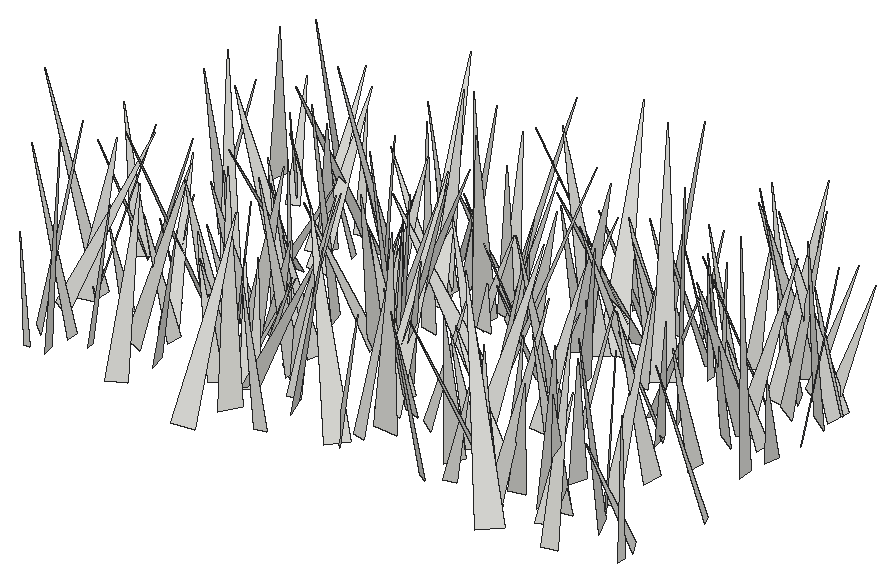
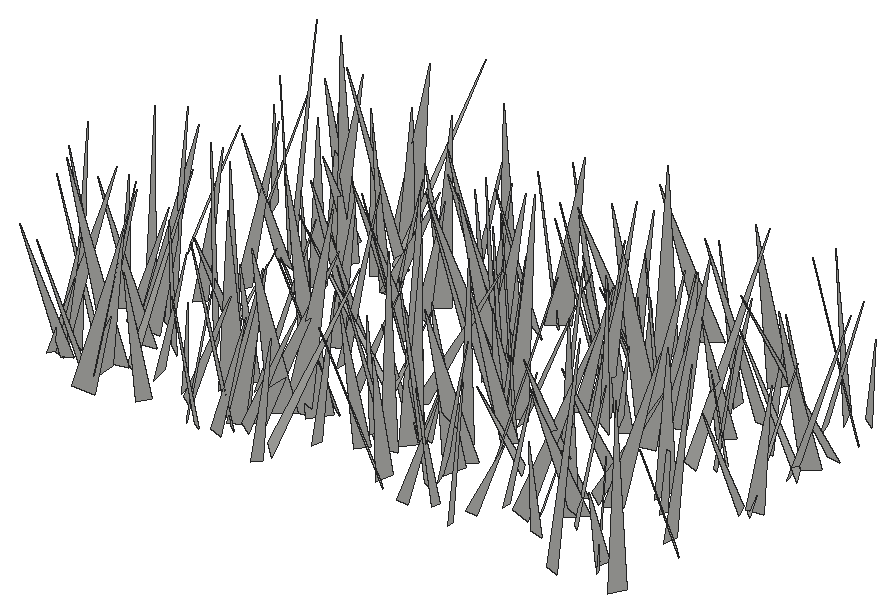
# SketchUp Ruby script. Lengths in inches.
U = 1.inch
M = Sketchup.active_model
def pt(a) = Geom::Point3d.new(a.map { |v| v * U })
def face(e, loops, mat)
  f = e.add_face(loops[0].map { |a| pt(a) })
  loops[1..].each { |l| e.add_face(l.map { |a| pt(a) }).erase! }
  f.material = f.back_material = mat if mat
  f
end
# faces: each face lists its corners as indices into pts; further lists are holes
def faces(e, pts, list, mat = nil) = list.each { |f| face(e, (f[0].is_a?(Array) ? f : [f]).map { |l| l.map { |i| pts[i] } }, mat) }
# xy, xz, yz: faces in a plane at the given z, y or x. An outline is a flat list of corners, or four numbers for a rectangle; further outlines are holes
def ring(l) = l.size == 4 ? [[l[0], l[1]], [l[2], l[1]], [l[2], l[3]], [l[0], l[3]]] : l.each_slice(2).to_a
def flat(e, list, mat, &to3) = list.each { |f| face(e, (f[0].is_a?(Array) ? f : [f]).map { |l| ring(l).map { |u, v| to3.(u, v) } }, mat) }
def xy(e, z, list, mat = nil) = flat(e, list, mat) { |x, y| [x, y, z] }
def xz(e, y, list, mat = nil) = flat(e, list, mat) { |x, z| [x, y, z] }
def yz(e, x, list, mat = nil) = flat(e, list, mat) { |y, z| [x, y, z] }
def lines(e, pts, list) = list.each { |a, b| e.add_line(pt(pts[a]), pt(pts[b])) }
# prism: a flat outline (further loops are holes) pulled along v
def prism(e, loops, v, mat = nil)
  f = face(e, loops, mat); d = Geom::Vector3d.new(v.map { |x| x * U })
  f.pushpull(f.normal.samedirection?(d) ? d.length : -d.length)
end
def box(e, o, s, mat = nil) = prism(e, [[o, [o[0] + s[0], o[1], o[2]], [o[0] + s[0], o[1] + s[1], o[2]], [o[0], o[1] + s[1], o[2]]]], [0, 0, s[2]], mat)
def at(x, y, z, deg = 0) = Geom::Transformation.translation(pt([x, y, z])) * Geom::Transformation.rotation(ORIGIN, Z_AXIS, deg.degrees)
def axes(o, x, y, z) = Geom::Transformation.new([*x, 0, *y, 0, *z, 0, *pt(o).to_a, 1])
def part(name) = M.definitions.add(name)
# library, detail: a bought-in or finely detailed component or shape, given as its bounding box
def library(name, o, s) = part(name).tap { |d| box(d.entities, o, s) }
def detail(e, o, s) = box(e.add_group.entities, o, s)
def put(e, d, t, mat = nil) = e.add_instance(d, t).tap { |i| i.material = mat if mat }
def group(e, t, mat = nil) = e.add_group.tap { |g| g.transformation = t; g.material = mat if mat }.entities
root = M.entities
c1 = part("fur_instance\#9")
p = [[0.8125,0,1.79],[0.67,-0.02,1.48],[0,-0.11,0],[0,0.11,0]]
faces(c1.entities,p,[[0,1,2,3]])
put(root,c1,axes([470.13,224.69,-21.66],[-2.04424,6.85145,0.72305],[6.79433,2.1298,-0.97223],[1.1412,-0.40704,7.08351]))
put(root,c1,axes([456.1,226.65,-21.66],[1.10778,3.32388,1.25845],[3.28018,-1.46364,0.97838],[-1.36832,-0.8177,3.36424]))
put(root,c1,axes([491.39,229.9,-21.66],[-5.30348,-5.59312,0.1785],[-5.55783,5.29332,0.73008],[0.65218,-0.37354,7.67313]))
put(root,c1,axes([474.1875,227.32,-21.66],[-0.90978,-4.59674,2.27002],[-5.08569,0.51819,-0.98893],[-0.64715,2.39002,4.58036]))
put(root,c1,axes([463.36,226.53,-21.66],[-4.06355,5.05875,1.67662],[5.05755,4.32523,-0.79246],[1.68023,-0.78477,6.44014]))
put(root,c1,axes([493.18,226.52,-21.66],[-5.00695,6.61488,0.9269],[6.67749,4.92855,0.89773],[-0.16413,-1.27989,8.24744]))
put(root,c1,axes([492.35,227.49,-21.66],[-0.54447,5.56352,1.73211],[5.79599,0.33809,0.73596],[-0.59958,-1.78391,5.54144]))
put(root,c1,axes([457.49,227.05,-21.66],[-6.13991,-1.94187,2.86824],[-2.65031,6.39227,-1.34568],[2.23013,2.25037,6.2975]))
put(root,c1,axes([501.75,230.24,-21.66],[-4.09527,-2.1175,0.66115],[-1.87882,4.04889,1.32991],[1.17939,-0.90267,4.41434]))
put(root,c1,axes([478.91,229.25,-21.66],[3.62429,3.41254,1.71474],[3.78655,-3.51895,-1.00013],[-0.49783,-1.92166,4.87654]))
put(root,c1,axes([495.22,231.08,-21.66],[5.27759,-3.33069,0.22963],[-3.2336,-5.20637,-1.19863],[-0.83073,-0.89406,6.12452]))
put(root,c1,axes([485.89,228.88,-21.66],[-3.65286,-4.07637,1.60167],[-4.37583,3.48496,-1.11027],[0.18514,1.94004,5.3598]))
put(root,c1,axes([497.68,226.82,-21.66],[0.68594,6.83231,0.78357],[6.74689,-0.82108,1.2531],[-1.33188,-0.64057,6.75135]))
put(root,c1,axes([471.09,228.24,-21.66],[-7.16118,3.19135,1.99245],[3.1192,7.43157,-0.69239],[2.1036,-0.15533,7.80947]))
put(root,c1,axes([487.46,229.67,-21.66],[2.40925,-3.29701,1.00546],[-3.44676,-2.29271,0.74099],[0.03277,1.24857,4.01568]))
put(root,c1,axes([502.13,228.43,-21.66],[-4.48133,-0.60292,1.35721],[-0.97091,4.45413,-1.22715],[1.12377,1.44397,4.35201]))
put(root,c1,axes([463.83,230.01,-21.66],[5.32416,0.8497,1.29821],[1.01973,-5.41351,-0.63884],[-1.1694,-0.85204,5.35356]))
put(root,c1,axes([494.05,231.1875,-21.66],[6.83248,-2.68093,1.04491],[-2.55055,-6.88917,-0.99801],[-1.33189,-0.56029,7.27146]))
put(root,c1,axes([498.56,231.05,-21.66],[-6.30807,-3.21691,2.7037],[-2.95993,6.86307,1.25992],[2.98285,0.00727,6.96799]))
put(root,c1,axes([491.66,231.125,-21.66],[2.32363,-4.81619,0.47979],[-4.81966,-2.25368,0.71896],[0.44354,0.74187,5.29887]))
put(root,c1,axes([457.63,229.3,-21.66],[-6.22819,-1.34042,0.61243],[-1.44458,6.07908,-1.38568],[0.29149,1.48668,6.21828]))
put(root,c1,axes([478.98,229.01,-21.66],[-5.24663,5.623,0.95369],[5.70188,5.20042,0.70642],[0.12741,-1.17997,7.65808]))
put(root,c1,axes([495.56,230.88,-21.66],[0.0044,-6.27087,2.13822],[-6.5778,-0.25997,-0.7489],[-0.79272,2.12236,6.226]))
put(root,c1,axes([455.375,228.73,-21.66],[4.64173,5.41011,1.53464],[5.42173,-4.8336,0.64123],[-1.49305,-0.73288,7.09956]))
put(root,c1,axes([459.18,229.15,-21.66],[-4.14484,-0.82966,2.07391],[-1.4546,4.32013,-1.17886],[1.69516,1.67847,4.05935]))
put(root,c1,axes([491.34,229.2,-21.66],[2.79902,6.82497,1.56007],[7.00009,-2.70115,-0.74237],[0.11309,-1.72399,7.33919]))
put(root,c1,axes([486.125,231.82,-21.66],[4.8862,-3.80667,1.31151],[-3.74132,-5.05482,-0.73291],[-1.48774,0.20937,6.1505]))
put(root,c1,axes([474.12,230.89,-21.66],[6.26752,1.77798,1.53658],[2.00319,-6.33057,-0.84565],[-1.22862,-1.25168,6.45971]))
put(root,c1,axes([495.37,228.99,-21.66],[-3.3116,2.69695,0.72945],[2.42136,3.33487,-1.33716],[1.39378,0.61437,4.05614]))
put(root,c1,axes([468.21,230.36,-21.66],[-1.43576,4.62376,1.24523],[4.74317,1.1948,1.0324],[-0.65727,-1.47798,4.73019]))
put(root,c1,axes([480.35,232.14,-21.66],[1.05516,-7.50337,2.43147],[-7.87164,-0.84629,0.8044],[0.49989,2.51181,7.53438]))
put(root,c1,axes([470.29,231.2,-21.66],[5.56558,-2.4926,0.3103],[-2.49513,-5.39934,1.38077],[0.28926,1.38533,5.93988]))
put(root,c1,axes([467.14,232.96,-21.66],[-3.93498,0.71077,2.15609],[1.47172,4.08376,1.33974],[1.72857,-1.85895,3.76754]))
put(root,c1,axes([461.14,230.93,-21.66],[2.20928,6.37096,1.50715],[6.50914,-1.9672,-1.22586],[0.70121,-1.81177,6.63078]))
put(root,c1,axes([473.26,231.86,-21.66],[-1.45732,3.49071,1.72371],[3.67662,1.83923,-0.61623],[1.28012,-1.30851,3.73217]))
put(root,c1,axes([462.875,232.95,-21.66],[-4.43499,0.78648,1.49873],[1.10021,4.53377,0.87655],[1.28619,-1.16631,4.41807]))
put(root,c1,axes([470.23,230.9375,-21.66],[-1.23415,4.06964,0.18802],[4.01431,1.18128,0.78126],[-0.69473,-0.40381,4.18028]))
put(root,c1,axes([489.87,232.67,-21.66],[-1.04898,-5.12431,2.12616],[-5.35306,1.50327,0.98203],[1.45734,1.83333,5.13756]))
put(root,c1,axes([497.5,232.68,-21.66],[5.0794,2.90769,2.21904],[3.29641,-5.28463,-0.62087],[-1.58507,-1.67247,5.81975]))
put(root,c1,axes([458.54,233.8,-21.66],[3.22144,-2.0672,0.86258],[-1.86043,-3.31076,-0.98626],[-1.24746,-0.40075,3.69841]))
put(root,c1,axes([489.88,232.375,-21.66],[-3.98181,3.20015,0.16473],[3.12043,3.81261,1.36007],[-0.7287,-1.16015,4.92402]))
put(root,c1,axes([489.4,232.01,-21.66],[-5.02924,-0.94611,0.83871],[-1.10156,4.96734,-1.00192],[0.62059,1.14984,5.01842]))
put(root,c1,axes([470.28,231.74,-21.66],[3.75823,0.40452,0.85087],[0.18545,-3.74836,0.96295],[-0.9237,0.89332,3.65522]))
put(root,c1,axes([470.07,231.92,-21.66],[-3.57041,1.71359,0.7726],[1.61509,3.64514,-0.62093],[0.96166,0.24019,3.91135]))
put(root,c1,axes([479.47,230.55,-21.66],[2.76869,6.15296,0.77217],[6.00563,-2.8712,1.34513],[-1.54517,-0.13446,6.61174]))
put(root,c1,axes([480.22,234.93,-21.66],[-0.97227,-5.54065,0.71566],[-5.53732,1.05209,0.62249],[0.741,0.5921,5.59077]))
put(root,c1,axes([468.65,232.81,-21.66],[3.29309,2.39527,0.08068],[2.3726,-3.23886,-0.68467],[0.3385,-0.60058,4.0141]))
put(root,c1,axes([486.05,233.79,-21.66],[1.60844,-3.68609,1.55705],[-3.78668,-1.94455,-0.69177],[-1.29334,1.10916,3.96179]))
put(root,c1,axes([493.79,234.54,-21.66],[4.8037,-2.51399,0.9877],[-2.43404,-4.90267,-0.64073],[-1.17095,-0.12226,5.38379]))
put(root,c1,axes([465.04,234.74,-21.66],[3.86572,-4.28586,2.24353],[-4.19582,-4.39988,-1.17556],[-2.40771,0.7863,5.6507]))
put(root,c1,axes([471.23,234.42,-21.66],[-6.84332,-0.22544,2.15666],[-0.013,7.14388,0.70553],[2.16837,-0.66867,6.81058]))
put(root,c1,axes([454.86,231.66,-21.66],[2.4491,6.4359,0.09226],[6.32974,-2.3903,-1.28384],[1.16776,-0.54137,6.7654]))
put(root,c1,axes([455.2,233.52,-21.66],[2.82826,-4.43632,2.67471],[-5.15951,-2.68482,1.00262],[-0.46309,2.81866,5.16476]))
put(root,c1,axes([466.21,234.82,-21.66],[-4.16703,-2.76107,2.92288],[-2.78486,5.0182,0.77013],[2.90022,0.85149,4.93909]))
put(root,c1,axes([467.42,234.57,-21.66],[6.54433,-2.87567,1.841],[-3.10892,-6.66403,0.64215],[-1.41189,1.3447,7.11937]))
put(root,c1,axes([470.91,234.13,-21.66],[3.79421,5.57197,1.64798],[5.81056,-3.63804,-1.07735],[0.00109,-1.96889,6.65448]))
put(root,c1,axes([461.38,237.88,-21.66],[-3.81436,-7.20009,0.2192],[-7.12697,3.80817,1.069],[1.0467,-0.30859,8.07762]))
put(root,c1,axes([482.01,234.24,-21.66],[2.56604,4.25646,1.10853],[4.39439,-2.42581,-0.85772],[0.18887,-1.38883,4.89555]))
put(root,c1,axes([455.83,234.56,-21.66],[-7.51977,-1.08655,0.44758],[-1.14316,7.43533,-1.15625],[0.27218,1.20961,7.50937]))
put(root,c1,axes([478.6,236.2,-21.66],[3.4747,-4.84053,2.29693],[-4.84614,-4.00697,-1.11322],[-2.28507,1.13736,5.85363]))
put(root,c1,axes([503.1,235.72,-21.66],[-4.74174,-2.50609,0.51828],[-2.55748,4.67952,-0.77105],[0.09149,0.92453,5.30754]))
put(root,c1,axes([470.41,234.95,-21.66],[4.17066,5.06918,1.33611],[5.23853,-4.09478,-0.81653],[-0.19883,-1.55319,6.51339]))
put(root,c1,axes([461.78,233.76,-21.66],[-3.2921,4.67046,0.35788],[4.62081,3.30978,-0.68745],[0.76768,0.10645,5.67261]))
put(root,c1,axes([478.07,237.11,-21.66],[6.05752,-0.57817,0.88939],[-0.39,-6.0087,-1.2499],[-0.9865,-1.17476,5.9553]))
put(root,c1,axes([459.88,237.24,-21.66],[-2.01295,-3.23513,0.63988],[-3.06607,2.112,1.03257],[1.21439,-0.03018,3.66768]))
put(root,c1,axes([467.22,237.16,-21.66],[2.01974,-4.62687,0.27657],[-4.52399,-1.90214,1.21619],[1.00891,0.73329,4.89981]))
put(root,c1,axes([459.48,236.53,-21.66],[4.05743,2.55482,1.17911],[2.80714,-3.81746,-1.3882],[-0.19333,-1.81108,4.58942]))
put(root,c1,axes([471.05,236.77,-21.66],[3.41803,-2.18502,2.15563],[-1.95303,-4.03718,-0.99543],[-2.36786,0.1758,3.93273]))
put(root,c1,axes([465.02,237.84,-21.66],[2.93992,-5.13493,1.13143],[-5.01799,-3.12719,-1.15379],[-1.5708,0.37938,5.8034]))
put(root,c1,axes([464.36,237.07,-21.66],[0.87067,-3.63818,0.96208],[-3.64876,-1.05785,-0.69825],[-0.92116,0.75142,3.67517]))
put(root,c1,axes([455.3125,234.68,-21.66],[5.06961,3.19969,0.78256],[3.08145,-5.11429,0.94868],[-1.16407,0.39664,5.91937]))
put(root,c1,axes([497.24,233.55,-21.66],[1.20703,6.81999,0.05967],[6.70849,-1.19813,1.23829],[-1.22962,0.158,6.81439]))
put(root,c1,axes([469.2,237.79,-21.66],[-5.69321,-2.11736,2.09192],[-1.78965,6.04293,1.24584],[2.37833,-0.52131,5.94506]))
put(root,c1,axes([478.99,234.03,-21.66],[-1.14842,8.02715,0.79991],[8.02073,1.22255,-0.75306],[0.86188,-0.68125,8.07384]))
put(root,c1,axes([478,235.87,-21.66],[7.83085,1.1219,1.78667],[1.00117,-8.02181,0.64907],[-1.85702,0.40616,7.88414]))
put(root,c1,axes([478.03,235.95,-21.66],[2.88835,4.68484,1.93004],[4.79823,-3.24275,0.69058],[-1.62782,-1.24585,5.46016]))
put(root,c1,axes([469.86,236.3,-21.66],[-2.9661,5.6248,1.68099],[5.86235,2.73802,1.18234],[-0.31135,-2.03143,6.24805]))
put(root,c1,axes([497.25,237.65,-21.66],[-5.83631,0.9789,1.84731],[1.28037,6.00401,0.86359],[1.65271,-1.19453,5.85448]))
put(root,c1,axes([476.66,238.07,-21.66],[6.37942,2.61315,2.43113],[3.05762,-6.56979,-0.96169],[-1.84118,-1.85616,6.82648]))
put(root,c1,axes([473.53,239.96,-21.66],[0.50064,-7.21064,0.91051],[-7.21991,-0.3887,0.89157],[0.83387,0.96363,7.17281]))
put(root,c1,axes([467.76,237.01,-21.66],[-4.02809,-0.22088,0.67447],[-0.39433,3.92835,-1.06856],[0.59008,1.11738,3.89005]))
put(root,c1,axes([488.08,239.91,-21.66],[3.42227,-3.49613,0.30492],[-3.40506,-3.41104,-0.89344],[-0.84941,-0.41195,4.81005]))
put(root,c1,axes([484.82,236.45,-21.66],[0.10942,6.44965,1.02032],[6.44115,0.06102,-1.07648],[1.07264,-1.02435,6.36012]))
put(root,c1,axes([468.54,237.52,-21.66],[2.01081,5.29668,2.07869],[5.40677,-2.46554,1.0522],[-1.77275,-1.51176,5.56697]))
put(root,c1,axes([454.66,240.42,-21.66],[-3.71629,-3.62879,0.54604],[-3.4741,3.72939,1.13989],[1.18191,-0.44788,5.0675]))
put(root,c1,axes([472.95,240.23,-21.66],[-5.60277,-1.40853,0.55452],[-1.25772,5.51462,1.29985],[0.84237,-1.13469,5.62898]))
put(root,c1,axes([474.89,239.37,-21.66],[5.41416,-4.66063,0.97473],[-4.76032,-5.26587,1.26282],[0.1044,1.59183,7.03135]))
put(root,c1,axes([487.88,238.04,-21.66],[-0.68675,5.73435,1.62653],[5.78722,1.03346,-1.2],[1.42703,-1.4315,5.64928]))
put(root,c1,axes([498.39,240.54,-21.66],[4.51587,-1.82573,1.61231],[-1.49442,-4.75873,-1.20297],[-1.92343,-0.58918,4.72009]))
put(root,c1,axes([484.13,237.84,-21.66],[4.06792,5.19434,1.22411],[5.14399,-4.22635,0.83955],[-1.42088,-0.42943,6.54403]))
put(root,c1,axes([454.54,239.96,-21.66],[-2.06507,4.56305,1.47225],[4.79287,1.92061,0.77009],[-0.13147,-1.65628,4.94903]))
put(root,c1,axes([474.97,239.45,-21.66],[7.79072,-0.23447,0.87822],[-0.35324,-7.76347,1.06082],[-0.83754,1.09323,7.72172]))
put(root,c1,axes([486.36,241.35,-21.66],[-6.02473,-0.71032,1.74625],[-0.51818,6.24626,0.75302],[1.81257,-0.57532,6.01954]))
put(root,c1,axes([494.53,241.78,-21.66],[5.27182,0.13194,1.25121],[0.40362,-5.28245,-1.14356],[-1.19165,-1.2055,5.14798]))
put(root,c1,axes([474.9,240.03,-21.66],[-4.32916,0.66549,1.27706],[0.40908,4.44763,-0.93094],[1.38073,0.76884,4.27993]))
put(root,c1,axes([474.12,240.78,-21.66],[-5.98871,-2.33617,1.80164],[-2.60473,6.10133,-0.74665],[1.38529,1.37273,6.38474]))
put(root,c1,axes([472.31,241.68,-21.66],[5.33637,4.77614,2.80857],[5.34994,-5.45601,-0.88678],[-1.44141,-2.56842,7.10647]))
put(root,c1,axes([469.09,241.26,-21.66],[-6.68963,-2.36331,2.10659],[-2.62997,6.88987,-0.62215],[1.76244,1.31094,7.06748]))
put(root,c1,axes([479.42,242.25,-21.66],[-6.11827,1.22354,0.04324],[1.20265,5.96505,1.37981],[-0.22923,-1.36132,6.08493]))
put(root,c1,axes([455.33,240.36,-21.66],[3.79033,1.52401,0.8214],[1.29616,-3.80865,1.0854],[-1.14773,0.73179,3.93842]))
put(root,c1,axes([489.63,240.12,-21.66],[2.15657,3.40289,0.33157],[3.29952,-2.17412,0.8525],[-0.89598,0.18416,3.93747]))
put(root,c1,axes([494.66,241.98,-21.66],[-3.19994,-2.12817,0.10035],[-2.08753,3.09569,-0.91527],[-0.42587,0.81635,3.73243]))
put(root,c1,axes([483.8,243.17,-21.66],[-1.02707,-3.52995,0.46815],[-3.49734,0.90838,-0.82343],[-0.66956,0.66999,3.58293]))
put(root,c1,axes([458.94,243.56,-21.66],[3.4639,-0.21189,1.20284],[0.06017,-3.58323,-0.80448],[-1.21988,-0.7784,3.37584]))
put(root,c1,axes([501.53,244.22,-21.66],[3.7269,-2.05729,0.24824],[-1.97365,-3.67974,-0.86491],[-0.63149,-0.64103,4.16823]))
put(root,c1,axes([501.33,241.83,-21.66],[-7.33304,-1.55705,2.53328],[-2.07568,7.50758,-1.39398],[2.1292,1.95633,7.36578]))
put(root,c1,axes([497.77,244.29,-21.66],[-3.27673,-6.38483,2.25273],[-6.55108,3.62196,0.73666],[1.71005,1.64109,7.13865]))
put(root,c1,axes([462.99,242.83,-21.66],[4.12414,-1.44643,0.07491],[-1.4095,-3.95608,1.21201],[0.33327,1.1677,4.19901]))
put(root,c1,axes([486.26,244.59,-21.66],[6.1777,-0.38175,1.16241],[-0.13775,-6.16226,-1.29169],[-1.21571,-1.24165,6.0532]))
put(root,c1,axes([498.44,245.61,-21.66],[1.25653,-6.81976,0.6894],[-6.81087,-1.32116,-0.65555],[-0.77223,0.55558,6.90349]))
put(root,c1,axes([460.31,241.7,-21.66],[-6.55915,2.85076,0.80174],[2.70921,6.56329,-1.17278],[1.19574,0.76707,7.05506]))
put(root,c1,axes([472.05,242.58,-21.66],[-0.35457,5.93898,1.63328],[6.05839,0.63143,-0.98081],[1.11129,-1.54746,5.86815]))
put(root,c1,axes([463.4,244.8,-21.66],[-2.21504,-4.22644,0.02495],[-4.06696,2.12371,-1.31133],[-1.15036,0.62998,4.58799]))
put(root,c1,axes([500.15,245.09,-21.66],[-3.89042,0.9571,1.21715],[1.27935,3.84105,1.06884],[0.87221,-1.36496,3.86121]))
put(root,c1,axes([474.51,243.8,-21.66],[1.78909,6.44129,2.50482],[6.73985,-2.19865,0.83993],[-1.52927,-2.15428,6.63216]))
put(root,c1,axes([461.87,244.96,-21.66],[-5.02266,3.34128,1.54054],[3.64584,4.87057,1.32283],[0.49523,-1.96924,5.88569]))
put(root,c1,axes([476.65,246.65,-21.66],[7.55718,-3.05255,1.8054],[-2.7949,-7.74218,-1.39129],[-2.18313,-0.65505,8.03077]))
put(root,c1,axes([481.8,242.32,-21.66],[5.80303,5.01805,0.27093],[4.96083,-5.78629,0.91567],[-0.80277,0.51711,7.61693]))
put(root,c1,axes([492.18,243.89,-21.66],[4.56042,0.58445,0.815],[0.35248,-4.48653,1.24501],[-0.93891,1.15443,4.42595]))
put(root,c1,axes([456.45,246.05,-21.66],[-5.67591,-0.59927,2.29984],[-0.30227,6.08824,0.84044],[2.35734,-0.66225,5.64524]))
put(root,c1,axes([493.87,244.5625,-21.66],[-6.60957,-3.13791,3.29203],[-3.79035,7.01015,-0.92809],[2.51341,2.31982,7.25752]))
put(root,c1,axes([488.53,246.95,-21.66],[-5.81258,-1.56867,1.18702],[-1.32265,5.85738,1.26392],[1.45614,-0.94136,5.88637]))
put(root,c1,axes([470.77,245.8,-21.66],[-7.3033,-3.33888,1.09507],[-3.45877,7.27632,-0.88176],[0.61989,1.26191,7.98178]))
put(root,c1,axes([463.27,247.67,-21.66],[5.23311,-3.59302,0.50013],[-3.53385,-5.24745,-0.7222],[-0.81967,-0.31597,6.30664]))
put(root,c1,axes([483.375,247.37,-21.66],[5.39011,-5.98506,0.75501],[-6.02641,-5.29691,1.03406],[0.27067,1.25142,7.9878]))
put(root,c1,axes([479.37,246.98,-21.66],[3.73813,0.01426,0.67221],[0.17612,-3.68545,-0.90117],[-0.64889,-0.91811,3.62791]))
put(root,c1,axes([476.63,246.17,-21.66],[-0.2038,-3.57727,1.86557],[-3.68837,0.92217,1.36537],[1.63497,1.63446,3.31273]))
put(root,c1,axes([479.48,246.96,-21.66],[-3.75562,-3.58045,0.3486],[-3.58145,3.67402,-0.84892],[-0.33818,0.85312,5.11895]))
put(root,c1,axes([489.34,246.4375,-21.66],[1.31397,-3.56018,1.31098],[-3.78942,-1.16427,0.63629],[0.18405,1.44556,3.7412]))
put(root,c1,axes([484.41,246.98,-21.66],[3.50873,2.55931,1.93983],[3.03472,-3.58228,-0.76287],[-1.05048,-1.80039,4.27543]))
put(root,c1,axes([469.1875,244.78,-21.66],[3.38601,2.0667,0.33408],[1.88033,-3.28152,1.24252],[-0.92044,0.89903,3.76728]))
put(root,c1,axes([476.36,245.48,-21.66],[-0.98772,3.5916,0.11089],[3.35733,0.88143,1.35606],[-1.28071,-0.45933,3.46934]))
put(root,c1,axes([476.99,245.92,-21.66],[1.25442,7.48082,2.76942],[7.81491,-1.71475,1.09211],[-1.59984,-2.51056,7.50623]))
put(root,c1,axes([477.25,248.06,-21.66],[0.11264,-6.37998,1.60761],[-6.5012,0.13924,1.0081],[1.01142,1.60553,6.30084]))
put(root,c1,axes([462.07,248.4,-21.66],[-3.11173,-3.4795,0.92655],[-3.33661,3.24675,0.98692],[1.3537,0.0043,4.56244]))
put(root,c1,axes([482.78,246.28,-21.66],[3.70587,4.25797,0.60198],[4.28884,-3.60158,-0.92773],[0.31394,-1.06043,5.56805]))
put(root,c1,axes([495.72,246.46,-21.66],[2.53366,4.26731,1.78001],[4.34271,-2.89305,0.75426],[-1.5872,-1.10369,4.90515]))
put(root,c1,axes([496.5,249.8125,-21.66],[-4.09518,-5.32392,0.52178],[-5.17841,4.11019,1.29512],[1.34181,-0.38619,6.5907]))
put(root,c1,axes([465.73,249.42,-21.66],[-1.54524,-6.7658,0.51217],[-6.71547,1.44992,-1.10738],[-0.96994,0.74015,6.85109]))
put(root,c1,axes([464.27,245.33,-21.66],[-1.14169,6.19263,0.48775],[6.13199,1.20279,-0.91762],[0.99261,-0.30768,6.22978]))
put(root,c1,axes([478.04,247.32,-21.66],[3.54049,4.95211,1.34575],[5.12044,-3.30078,-1.32493],[0.33991,-1.85767,5.94164]))
put(root,c1,axes([467.2,248.93,-21.66],[-4.25466,-1.2014,1.34721],[-0.93808,4.41863,0.97784],[1.54219,-0.62673,4.31153]))
put(root,c1,axes([484.75,247.86,-21.66],[1.79805,-6.87497,3.712],[-7.43664,-2.674,-1.35027],[-2.39594,3.14033,6.97674]))
put(root,c1,axes([497.25,247.03,-21.66],[1.23681,5.98503,1.54047],[6.1022,-0.934,-1.27052],[0.97821,-1.7408,5.97797]))
put(root,c1,axes([478.81,248.83,-21.66],[3.21186,-3.52218,0.8528],[-3.62385,-3.13,0.72104],[-0.02677,1.11644,4.71189]))
put(root,c1,axes([464.93,248.25,-21.66],[-3.69691,-1.68274,0.52652],[-1.75981,3.59718,-0.85985],[0.10916,1.00233,3.96981]))
put(root,c1,axes([485.88,250.58,-21.66],[-1.10699,-6.38687,0.31821],[-6.26084,1.01671,-1.37367],[-1.30201,0.54128,6.33487]))
put(root,c1,axes([501.52,247.23,-21.66],[-4.45958,-2.36263,3.46386],[-3.3219,5.07642,-0.81428],[2.55838,2.47306,4.98064]))
put(root,c1,axes([500.88,249.76,-21.66],[-3.13728,-6.42445,2.27927],[-6.51063,3.56742,1.09378],[2.01998,1.52023,7.06539]))
put(root,c1,axes([455.16,246.9375,-21.66],[3.04107,3.48011,0.59696],[3.3547,-3.09349,0.94446],[-1.10161,0.1866,4.52408]))
put(root,c1,axes([472.42,247.5625,-21.66],[-5.70861,3.53079,2.01517],[3.32922,6.05385,-1.17592],[2.33318,0.00055,6.60847]))
put(root,c1,axes([481.35,250.2,-21.66],[4.6906,-0.13116,1.94102],[0.35682,-4.92253,-1.19491],[-1.91244,-1.24013,4.53774]))
put(root,c1,axes([487.46,250.02,-21.66],[3.16597,-2.82128,1.36449],[-2.73379,-3.43456,-0.75836],[-1.53229,0.2984,4.17228]))
put(root,c1,axes([487.93,250.64,-21.66],[2.45481,-4.16097,0.8917],[-4.06011,-2.59844,-0.9479],[-1.27449,0.26329,4.73722]))
put(root,c1,axes([472.73,248.48,-21.66],[-6.0397,-1.24718,1.08354],[-1.47294,5.92489,-1.39057],[0.74831,1.59618,6.00831]))
put(root,c1,axes([462.74,247.09,-21.66],[-1.71935,6.00909,0.23442],[5.94835,1.73522,-0.85232],[0.8839,0.01135,6.19184]))
put(root,c1,axes([472.59,246.35,-21.66],[-4.41357,6.91206,0.00056],[6.86097,4.38103,-0.99489],[0.83882,0.53496,8.14041]))
put(root,c1,axes([472.5,250.1,-21.66],[-2.78435,-5.66723,3.39056],[-5.97834,3.72634,1.319],[2.80584,2.3158,6.17497]))
put(root,c1,axes([486.87,251.38,-21.66],[-3.71631,2.59474,2.95715],[3.6126,3.86147,1.15179],[1.55775,-2.76492,4.38373]))
put(root,c1,axes([489.99,247.78,-21.66],[-7.18499,4.19207,1.05141],[4.04317,7.24035,-1.23823],[1.52698,0.55406,8.22584]))
put(root,c1,axes([498.52,249.43,-21.66],[3.30058,6.51639,2.13105],[6.85171,-3.21879,-0.76942],[-0.24255,-2.25268,7.26396]))
put(root,c1,axes([494.46,249.5,-21.66],[-5.51822,-0.21879,0.79161],[-0.32668,5.51842,-0.75206],[0.75352,0.79022,5.4711]))
put(root,c1,axes([501.37,251.09,-21.66],[-7.04891,1.70289,1.4017],[1.92518,7.04086,1.12767],[1.07622,-1.44158,7.16347]))
put(root,c1,axes([492.04,250.01,-21.66],[-3.53666,-0.44387,1.07965],[-0.6619,3.59984,-0.68824],[0.96154,0.84544,3.49732]))
put(root,c1,axes([490.95,251.1,-21.66],[-2.05485,-3.90462,0.97999],[-3.96047,1.76344,-1.27819],[-0.72186,1.43981,4.22312]))
put(root,c1,axes([486.05,251.43,-21.66],[-2.14589,-4.13922,0.79032],[-4.13009,1.88974,-1.31675],[-0.83673,1.28775,4.4726]))
put(root,c1,axes([457.51,251.98,-21.66],[3.15596,1.30372,1.61225],[1.82364,-3.14251,-1.02861],[-0.98659,-1.6383,3.25603]))
put(root,c1,axes([470.65,251.66,-21.66],[3.7872,-0.0255,0.26622],[0.02172,-3.73751,-0.66706],[-0.26655,-0.66693,3.72808]))
put(root,c1,axes([483.1,252.7,-21.66],[-4.92734,-5.46841,0.2776],[-5.45988,4.87887,-0.80338],[-0.41255,0.74316,7.31688]))
put(root,c1,axes([501.12,251.26,-21.66],[-0.94166,-4.10224,1.61468],[-4.38512,0.70145,-0.77524],[-0.45421,1.73259,4.13692]))
put(root,c1,axes([498.1,251.3,-21.66],[-6.28358,-3.49392,1.76213],[-3.72095,6.36668,-0.64478],[1.21124,1.43309,7.16066]))
put(root,c1,axes([472.57,252.67,-21.66],[0.53786,-3.60504,0.14249],[-3.55289,-0.5543,-0.6129],[-0.62738,0.04841,3.59304]))
put(root,c1,axes([485.4375,248.42,-21.66],[-4.43994,6.98412,0.3729],[6.94517,4.45476,-0.74146],[0.82561,0.08476,8.24265]))
put(root,c1,axes([468.29,251.09,-21.66],[-1.80359,3.13263,0.44398],[3.00697,1.53819,1.36218],[-0.98418,-1.04117,3.34825]))
put(root,c1,axes([497.26,250.15,-21.66],[0.16612,7.76506,1.97129],[7.95416,0.07536,-0.96713],[0.95574,-1.97685,7.70638]))
put(root,c1,axes([463.5,250.61,-21.66],[0.00503,4.167,0.7042],[4.17874,-0.11,0.62111],[-0.63075,-0.69557,4.12045]))
put(root,c1,axes([468.43,253.01,-21.66],[4.23217,0.79223,1.75299],[1.35483,-4.23497,-1.35698],[-1.36567,-1.74623,4.08626]))
put(root,c1,axes([459.77,253.68,-21.66],[-3.5221,-6.63629,1.77015],[-6.5539,3.84233,1.36448],[2.0543,0.8804,7.38808]))
put(root,c1,axes([489.56,252.88,-21.66],[-3.13954,-2.86345,1.03549],[-2.74612,3.30524,0.81394],[1.31545,0.06589,4.17056]))
put(root,c1,axes([500.37,251.31,-21.66],[0.61438,4.77457,1.24038],[4.786,-0.27399,-1.3159],[1.1955,-1.35681,4.63059]))
put(root,c1,axes([475.31,250.98,-21.66],[-4.49774,2.41965,1.22715],[2.26445,4.65664,-0.88215],[1.49428,0.22634,5.03052]))
put(root,c1,axes([454.97,253.19,-21.66],[5.79339,-2.08626,1.56673],[-1.97661,-6.00002,-0.68061],[-1.70297,-0.13319,6.11985]))
put(root,c1,axes([496.99,253.95,-21.66],[1.49882,-6.76146,1.59023],[-6.75855,-1.79498,-1.262],[-1.60255,1.24632,6.80963]))
put(root,c1,axes([487.15,253.04,-21.66],[-0.77658,-4.10323,1.17838],[-4.23531,0.59015,-0.73621],[-0.53592,1.28194,4.11067]))
put(root,c1,axes([457.85,251,-21.66],[-3.33951,2.40161,0.05247],[2.31618,3.24301,-1.02031],[0.63702,0.79874,3.98485]))
put(root,c1,axes([497.44,251.3125,-21.66],[-6.80477,1.06742,0.77743],[0.9228,6.76292,-1.20833],[0.94457,1.0827,6.78117]))
put(root,c1,axes([493.25,252.62,-21.66],[3.51253,-2.51047,1.78394],[-2.89575,-3.6135,0.61652],[-1.0486,1.56939,4.2732]))
put(root,c1,axes([482.89,254.26,-21.66],[3.48904,-1.79502,0.75996],[-1.60226,-3.52839,-0.97792],[-1.11014,-0.54905,3.7999]))
put(root,c1,axes([488.62,253.11,-21.66],[2.69077,3.3772,1.27263],[3.60609,-2.57991,-0.77814],[-0.14558,-1.48455,4.24737]))
put(root,c1,axes([498.06,252.375,-21.66],[2.30047,4.4169,0.81433],[4.47004,-2.16262,-0.89782],[0.43686,-1.13065,4.89848]))
put(root,c1,axes([487.16,251.55,-21.66],[4.31579,6.0344,1.65644],[5.97789,-4.5707,1.07586],[-1.85004,-0.69181,7.34048]))
put(root,c1,axes([475.23,251.45,-21.66],[4.30738,5.01035,0.65824],[4.94004,-4.35705,0.83813],[-1.06435,0.05398,6.55397]))
